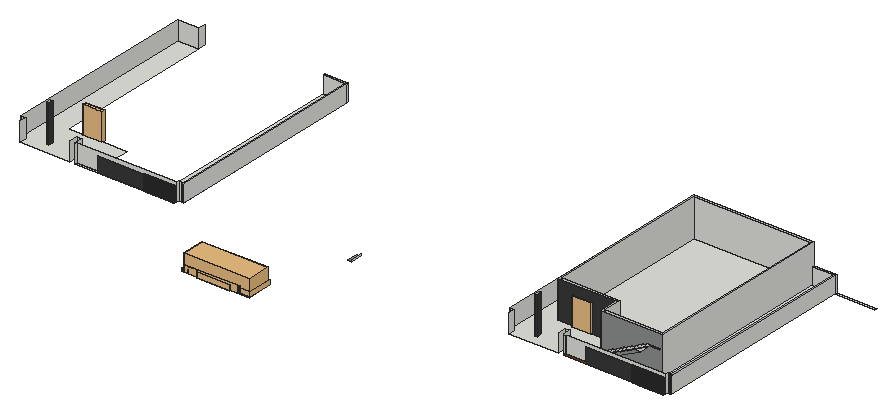
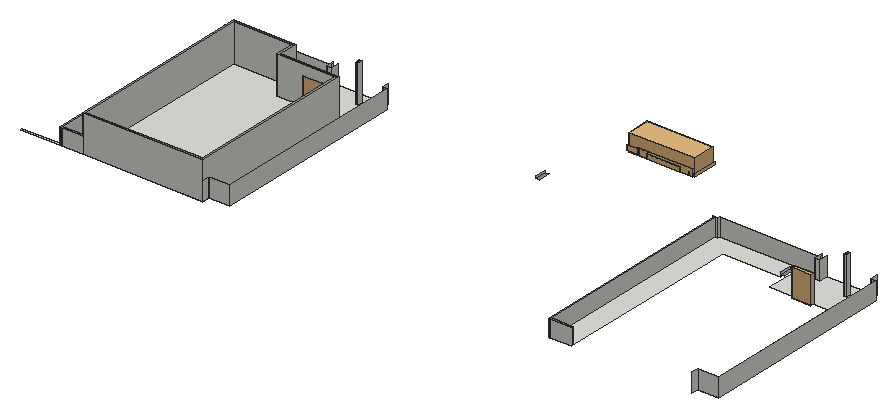
# SketchUp Ruby script. Lengths in inches.
U = 1.inch
M = Sketchup.active_model
def pt(a) = Geom::Point3d.new(a.map { |v| v * U })
def face(e, loops, mat)
  f = e.add_face(loops[0].map { |a| pt(a) })
  loops[1..].each { |l| e.add_face(l.map { |a| pt(a) }).erase! }
  f.material = f.back_material = mat if mat
  f
end
# faces: each face lists its corners as indices into pts; further lists are holes
def faces(e, pts, list, mat = nil) = list.each { |f| face(e, (f[0].is_a?(Array) ? f : [f]).map { |l| l.map { |i| pts[i] } }, mat) }
# xy, xz, yz: faces in a plane at the given z, y or x. An outline is a flat list of corners, or four numbers for a rectangle; further outlines are holes
def ring(l) = l.size == 4 ? [[l[0], l[1]], [l[2], l[1]], [l[2], l[3]], [l[0], l[3]]] : l.each_slice(2).to_a
def flat(e, list, mat, &to3) = list.each { |f| face(e, (f[0].is_a?(Array) ? f : [f]).map { |l| ring(l).map { |u, v| to3.(u, v) } }, mat) }
def xy(e, z, list, mat = nil) = flat(e, list, mat) { |x, y| [x, y, z] }
def xz(e, y, list, mat = nil) = flat(e, list, mat) { |x, z| [x, y, z] }
def yz(e, x, list, mat = nil) = flat(e, list, mat) { |y, z| [x, y, z] }
def lines(e, pts, list) = list.each { |a, b| e.add_line(pt(pts[a]), pt(pts[b])) }
# prism: a flat outline (further loops are holes) pulled along v
def prism(e, loops, v, mat = nil)
  f = face(e, loops, mat); d = Geom::Vector3d.new(v.map { |x| x * U })
  f.pushpull(f.normal.samedirection?(d) ? d.length : -d.length)
end
def box(e, o, s, mat = nil) = prism(e, [[o, [o[0] + s[0], o[1], o[2]], [o[0] + s[0], o[1] + s[1], o[2]], [o[0], o[1] + s[1], o[2]]]], [0, 0, s[2]], mat)
def at(x, y, z, deg = 0) = Geom::Transformation.translation(pt([x, y, z])) * Geom::Transformation.rotation(ORIGIN, Z_AXIS, deg.degrees)
def axes(o, x, y, z) = Geom::Transformation.new([*x, 0, *y, 0, *z, 0, *pt(o).to_a, 1])
def part(name) = M.definitions.add(name)
# library, detail: a bought-in or finely detailed component or shape, given as its bounding box
def library(name, o, s) = part(name).tap { |d| box(d.entities, o, s) }
def detail(e, o, s) = box(e.add_group.entities, o, s)
def put(e, d, t, mat = nil) = e.add_instance(d, t).tap { |i| i.material = mat if mat }
def group(e, t, mat = nil) = e.add_group.tap { |g| g.transformation = t; g.material = mat if mat }.entities
root = M.entities
M.materials.add("[Blacktop Old 02]").color = [143, 145, 145]
M.materials.add("[Color M07]").color = [58, 58, 58]
M.materials.add("[Wood Veneer 01]").color = [120, 70, 37]
M.materials.add("s600").color = [22, 22, 22]
c1 = library("door (1)",[38.93,25.48,0],[40,9.94,82.68])
c2 = library("Group\#542",[3.69,3.66,0],[191.53,68.02,49.26])
c3 = library("Group\#537",[0,0,0],[105.78,6.21,15.76])
c4 = library("Group\#518",[0,0.23,0],[177.37,78.25,22.11])
c5 = library("Group\#530",[0,0,0],[20.12,77.4,9.12])
c6 = library("Group\#533",[0,0,0],[37.78,78.39,15.5])
xy(root,5.875,[[1229.53,300.25,1232.01,301],[1232.72,300.25,1235.19,301],[1235.91,300.25,1238.38,301],[1239.1,300.25,1241.57,301],[1242.28,300.25,1244.76,301],
  [1245.47,300.25,1247.94,301],[1248.66,300.25,1251.13,301],[1251.85,300.25,1254.32,301],[1255.03,300.25,1257.51,301],[1258.22,300.25,1260.69,301],
  [1261.41,300.25,1263.88,301],[1280.53,300.25,1283.01,301],[1283.72,300.25,1286.19,301],[1286.85,300.25,1289.32,301],[1289.97,300.25,1292.44,301],
  [1293.1,300.25,1295.57,301],[1296.22,300.25,1298.69,301],[1299.35,300.25,1301.82,301],[1302.47,300.25,1304.94,301],[1305.6,300.25,1308.07,301],
  [1308.72,300.25,1311.19,301],[1311.85,300.25,1314.32,301],[1314.97,300.25,1317.44,301],[1318.1,300.25,1320.28,301],[2783.53,300.25,2786.01,301],
  [2786.72,300.25,2789.19,301],[2789.91,300.25,2792.38,301],[2793.1,300.25,2795.57,301],[2796.28,300.25,2798.76,301],[2799.47,300.25,2801.94,301],
  [2802.66,300.25,2805.13,301],[2805.85,300.25,2808.32,301],[2809.03,300.25,2811.51,301],[2812.22,300.25,2814.69,301],[2815.41,300.25,2817.88,301],
  [2818.6,300.25,2821.07,301],[2821.78,300.25,2824.26,301],[2824.97,300.25,2827.44,301],[2828.16,300.25,2830.63,301],[2831.35,300.25,2833.82,301],
  [2834.53,300.25,2837.01,301],[2837.72,300.25,2840.19,301],[2840.91,300.25,2843.38,301],[2844.1,300.25,2846.57,301],[2847.28,300.25,2849.76,301],
  [2850.47,300.25,2852.94,301],[2853.6,300.25,2856.07,301],[2856.72,300.25,2859.19,301],[2859.85,300.25,2862.32,301],[2862.97,300.25,2865.44,301],
  [2866.1,300.25,2868.57,301],[2869.22,300.25,2871.69,301],[2872.35,300.25,2874.82,301],[2875.47,300.25,2877.94,301],[2878.6,300.25,2881.07,301],
  [2881.72,300.25,2884.19,301],[2884.85,300.25,2887.03,301],[[823.45,301,982.13,301,982.13,327.09,998.26,327.09,998.26,308.75,1320.28,308.75,1320.28,315.3125,1328.59,315.3125,1328.59,969.375,1260.59,969.375,1260.59,371.33,1072.95,371.33,1072.95,335.33,1061.03,335.33,1061.03,431.33,983.8,431.33,983.8,440.27,922.05,440.27,922.05,431.33,874.71,431.33,874.71,952.09,808.46,952.09,808.46,321.97,823.45,321.97],[879.98,334.62,887.35,350.3]],[998.26,301,1320.28,308.75],[[2390.2,301,2548.88,301,2548.88,327.09,2565.01,327.09,2565.01,308.75,2887.03,308.75,2887.03,315.3125,2895.34,315.3125,2895.34,969.375,2827.34,969.375,2827.34,371.33,2639.7,371.33,2639.7,335.33,2627.78,335.33,2627.78,431.33,2550.55,431.33,2550.55,440.27,2488.8,440.27,2488.8,431.33,2441.46,431.33,2441.46,952.09,2375.21,952.09,2375.21,321.97,2390.2,321.97],[2446.73,334.62,2454.1,350.3]],
  [2565.01,301,2887.03,308.75],[1328.59,315.3125,1334.59,969.375],[2895.34,315.3125,2901.34,969.375],[2627.78,335.33,2627.78,431.33,2550.55,431.33,2550.55,440.27,2633.78,440.27,2633.78,379.21,2822.07,379.21,2822.07,970.67,2446.73,970.67,2446.73,440.27,2488.8,440.27,2488.8,431.33,2441.46,431.33,2441.46,975.9375,2827.34,975.9375,2827.34,371.33,2639.7,371.33,2639.7,335.33],[2633.78,379.21,2822.07,379.21,2822.07,970.67,2446.73,970.67,2446.73,440.27,2633.78,440.27],
  [1260.59,969.375,1328.59,975.9375],[1328.59,969.375,1334.59,975.9375],[2827.34,969.375,2895.34,975.9375],[2895.34,969.375,2901.34,975.9375],[2901.34,969.375,3027.59,975.9375]])
xy(root,11.875,[[1061.03,335.33,1073.03,371.33],[1847.4,335.33,1859.4,371.33],[2627.78,335.33,2639.78,371.33]],"[Blacktop Old 02]")
xz(root,300.25,[[1229.53,5.875,1232.01,54.66],[1232.72,5.875,1235.19,54.66],[1235.91,5.875,1238.38,54.66],[1239.1,5.875,1241.57,54.66],[1242.28,5.875,1244.76,54.66],
  [1245.47,5.875,1247.94,54.66],[1248.66,5.875,1251.13,54.66],[1251.85,5.875,1254.32,54.66],[1255.03,5.875,1257.51,54.66],[1258.22,5.875,1260.69,54.66],
  [1261.41,5.875,1263.88,54.66],[1280.53,5.875,1283.01,54.66],[1283.72,5.875,1286.19,54.66],[1286.85,5.875,1289.32,54.66],[1289.97,5.875,1292.44,54.66],
  [1293.1,5.875,1295.57,54.66],[1296.22,5.875,1298.69,54.66],[1299.35,5.875,1301.82,54.66],[1302.47,5.875,1304.94,54.66],[1305.6,5.875,1308.07,54.66],
  [1308.72,5.875,1311.19,54.66],[1311.85,5.875,1314.32,54.66],[1314.97,5.875,1317.44,54.66],[1318.1,5.875,1320.28,54.66],[2783.53,5.875,2786.01,54.66],
  [2786.72,5.875,2789.19,54.66],[2789.91,5.875,2792.38,54.66],[2793.1,5.875,2795.57,54.66],[2796.28,5.875,2798.76,54.66],[2799.47,5.875,2801.94,54.66],
  [2802.66,5.875,2805.13,54.66],[2805.85,5.875,2808.32,54.66],[2809.03,5.875,2811.51,54.66],[2812.22,5.875,2814.69,54.66],[2815.41,5.875,2817.88,54.66],
  [2818.6,5.875,2821.07,54.66],[2821.78,5.875,2824.26,54.66],[2824.97,5.875,2827.44,54.66],[2828.16,5.875,2830.63,54.66],[2831.35,5.875,2833.82,54.66],
  [2834.53,5.875,2837.01,54.66],[2837.72,5.875,2840.19,54.66],[2840.91,5.875,2843.38,54.66],[2844.1,5.875,2846.57,54.66],[2847.28,5.875,2849.76,54.66],
  [2850.47,5.875,2852.94,54.66],[2853.6,5.875,2856.07,54.66],[2856.72,5.875,2859.19,54.66],[2859.85,5.875,2862.32,54.66],[2862.97,5.875,2865.44,54.66],
  [2866.1,5.875,2868.57,54.66],[2869.22,5.875,2871.69,54.66],[2872.35,5.875,2874.82,54.66],[2875.47,5.875,2877.94,54.66],[2878.6,5.875,2881.07,54.66],
  [2881.72,5.875,2884.19,54.66],[2884.85,5.875,2887.03,54.66]],"[Color M07]")
xz(root,301,[[2887.03,5.875,2887.32,54.66]])
xz(root,301,[[1070.49,5.875,1216.78,54.66],[1219.26,5.875,1219.97,54.66],[1222.44,5.875,1223.16,54.66],[1225.63,5.875,1226.35,54.66],[1228.82,5.875,1229.53,54.66],
  [1232.01,5.875,1232.72,54.66],[1235.19,5.875,1235.91,54.66],[1238.38,5.875,1239.1,54.66],[1241.57,5.875,1242.28,54.66],[1244.76,5.875,1245.47,54.66],
  [1247.94,5.875,1248.66,54.66],[1251.13,5.875,1251.85,54.66],[1254.32,5.875,1255.03,54.66],[1257.51,5.875,1258.22,54.66],[1260.69,5.875,1261.41,54.66],
  [1263.88,5.875,1264.6,54.66],[1267.07,5.875,1267.78,54.66],[1270.26,5.875,1270.97,54.66],[1273.44,5.875,1274.16,54.66],[1276.63,5.875,1277.35,54.66],
  [1279.82,5.875,1280.53,54.66],[1317.44,5.875,1318.1,54.66],[2637.24,5.875,2783.53,54.66],[2786.01,5.875,2786.72,54.66],[2789.19,5.875,2789.91,54.66],
  [2792.38,5.875,2793.1,54.66],[2795.57,5.875,2796.28,54.66],[2798.76,5.875,2799.47,54.66],[2801.94,5.875,2802.66,54.66],[2805.13,5.875,2805.85,54.66],
  [2808.32,5.875,2809.03,54.66],[2811.51,5.875,2812.22,54.66],[2814.69,5.875,2815.41,54.66],[2817.88,5.875,2818.6,54.66],[2821.07,5.875,2821.78,54.66],
  [2824.26,5.875,2824.97,54.66],[2827.44,5.875,2828.16,54.66],[2830.63,5.875,2831.35,54.66],[2833.82,5.875,2834.53,54.66],[2837.01,5.875,2837.72,54.66],
  [2840.19,5.875,2840.91,54.66],[2843.38,5.875,2844.1,54.66],[2846.57,5.875,2847.28,54.66],[2849.76,5.875,2850.47,54.66],[2852.94,5.875,2853.6,54.66],
  [2856.07,5.875,2856.72,54.66],[2859.19,5.875,2859.85,54.66],[2862.32,5.875,2862.97,54.66],[2865.44,5.875,2866.1,54.66],[2868.57,5.875,2869.22,54.66],
  [2871.69,5.875,2872.35,54.66],[2874.82,5.875,2875.47,54.66],[2877.94,5.875,2878.6,54.66],[2881.07,5.875,2881.72,54.66],[2884.19,5.875,2884.85,54.66]],"[Color M07]")
xz(root,301,[[2565.01,5.875,2637.24,13.04]],"[Wood Veneer 01]")
xz(root,308.75,[[998.26,5.875,1320.28,62.25],[2565.01,5.875,2887.03,62.25]])
xz(root,315.3125,[[1320.28,5.875,1320.28,62.25,1334.59,62.25,1334.59,58.8125,1328.59,58.8125,1328.59,5.875],[1328.59,5.875,1334.59,58.8125],[2887.03,5.875,2887.03,62.25,2901.34,62.25,2901.34,58.8125,2895.34,58.8125,2895.34,5.875],[2895.34,5.875,2901.34,58.8125]])
xz(root,321.97,[[808.46,5.875,823.45,65.875],[2375.21,5.875,2390.2,65.875]])
xz(root,327.09,[[982.13,5.875,998.26,65.875],[2548.88,5.875,2565.01,65.875]])
xz(root,334.62,[[879.98,5.875,887.35,125.875],[2446.73,5.875,2454.1,125.875]],"[Color M07]")
xz(root,335.33,[[2627.78,5.875,2639.7,5.875,2783.78,77.875,2759.78,77.875,2759.78,71.875,2747.78,71.875,2747.78,65.875,2735.78,65.875,2735.78,59.875,2723.78,59.875,2723.78,53.875,2711.78,53.875,2711.78,47.875,2699.78,47.875,2699.78,41.875,2687.78,41.875,2687.78,35.875,2675.78,35.875,2675.78,29.875,2663.78,29.875,2663.78,23.875,2651.78,23.875,2651.78,17.875,2639.78,17.875,2639.78,11.875,2627.78,11.875]],"[Blacktop Old 02]")
xz(root,350.3,[[879.98,5.875,887.35,125.875],[2446.73,5.875,2454.1,125.875]])
xz(root,371.33,[[2639.7,5.875,2827.34,5.875,2827.34,125.875,2627.78,125.875,2627.78,11.875,2639.78,11.875,2639.78,17.875,2651.78,17.875,2651.78,23.875,2663.78,23.875,2663.78,29.875,2675.78,29.875,2675.78,35.875,2687.78,35.875,2687.78,41.875,2699.78,41.875,2699.78,47.875,2711.78,47.875,2711.78,53.875,2723.78,53.875,2723.78,59.875,2735.78,59.875,2735.78,65.875,2747.78,65.875,2747.78,71.875,2759.78,71.875,2759.78,77.875,2771.78,77.875,2771.78,83.875,2819.78,83.875,2819.78,77.875,2783.78,77.875]],"[Blacktop Old 02]")
xz(root,379.21,[[2633.78,5.875,2822.07,125.875]])
xz(root,431.33,[[2441.46,5.875,2488.8,5.875,2488.8,94.0625,2550.55,94.0625,2550.55,5.875,2627.78,5.875,2627.78,125.875,2441.46,125.875]],"[Color M07]")
xz(root,440.27,[[2446.73,5.875,2446.73,125.875,2633.78,125.875,2633.78,5.875,2550.55,5.875,2550.55,94.0625,2488.8,94.0625,2488.8,5.875]])
xz(root,952.09,[[808.46,5.875,874.71,65.875],[2375.21,5.875,2441.46,65.875]])
xz(root,969.375,[[1260.59,5.875,1328.59,58.8125],[1328.59,5.875,1334.59,58.8125],[2827.34,5.875,2895.34,58.8125],[2895.34,5.875,2901.34,58.8125]])
xz(root,970.67,[[2446.73,5.875,2822.07,125.875]])
xz(root,975.9375,[[1260.59,5.875,1328.59,58.8125],[1328.59,5.875,1334.59,58.8125],[2441.46,5.875,2827.34,125.875],[2827.34,5.875,2895.34,58.8125],[2895.34,5.875,2901.34,58.8125]])
yz(root,808.46,[[321.97,5.875,952.09,65.875]])
yz(root,823.45,[[301,5.875,321.97,65.875]])
yz(root,874.71,[[952.09,5.875,975.9375,65.875]])
yz(root,879.98,[[334.62,5.875,350.3,125.875]])
yz(root,887.35,[[334.62,5.875,350.3,125.875]],"[Color M07]")
yz(root,982.13,[[301,5.875,327.09,65.875]])
yz(root,998.26,[[301,5.875,308.75,62.25],[308.75,5.875,327.09,5.875,327.09,65.875,301,65.875,301,62.25,308.75,62.25]])
yz(root,1073.03,[[335.33,11.875,371.33,17.875]])
yz(root,1229.53,[[300.25,5.875,301,54.66]])
yz(root,1232.01,[[300.25,5.875,301,54.66]])
yz(root,1232.72,[[300.25,5.875,301,54.66]])
yz(root,1235.19,[[300.25,5.875,301,54.66]])
yz(root,1235.91,[[300.25,5.875,301,54.66]])
yz(root,1238.38,[[300.25,5.875,301,54.66]])
yz(root,1239.1,[[300.25,5.875,301,54.66]])
yz(root,1241.57,[[300.25,5.875,301,54.66]])
yz(root,1242.28,[[300.25,5.875,301,54.66]])
yz(root,1244.76,[[300.25,5.875,301,54.66]])
yz(root,1245.47,[[300.25,5.875,301,54.66]])
yz(root,1247.94,[[300.25,5.875,301,54.66]])
yz(root,1248.66,[[300.25,5.875,301,54.66]])
yz(root,1251.13,[[300.25,5.875,301,54.66]])
yz(root,1251.85,[[300.25,5.875,301,54.66]])
yz(root,1254.32,[[300.25,5.875,301,54.66]])
yz(root,1255.03,[[300.25,5.875,301,54.66]])
yz(root,1257.51,[[300.25,5.875,301,54.66]])
yz(root,1258.22,[[300.25,5.875,301,54.66]])
yz(root,1260.69,[[300.25,5.875,301,54.66]])
yz(root,1261.41,[[300.25,5.875,301,54.66]])
yz(root,1263.88,[[300.25,5.875,301,54.66]])
yz(root,1277.35,[[300.25,5.875,301,54.66]])
yz(root,1280.53,[[300.25,5.875,301,54.66]])
yz(root,1283.01,[[300.25,5.875,301,54.66]])
yz(root,1283.72,[[300.25,5.875,301,54.66]])
yz(root,1286.19,[[300.25,5.875,301,54.66]])
yz(root,1286.85,[[300.25,5.875,301,54.66]])
yz(root,1289.32,[[300.25,5.875,301,54.66]])
yz(root,1289.97,[[300.25,5.875,301,54.66]])
yz(root,1292.44,[[300.25,5.875,301,54.66]])
yz(root,1293.1,[[300.25,5.875,301,54.66]])
yz(root,1295.57,[[300.25,5.875,301,54.66]])
yz(root,1296.22,[[300.25,5.875,301,54.66]])
yz(root,1298.69,[[300.25,5.875,301,54.66]])
yz(root,1302.47,[[300.25,5.875,301,54.66]])
yz(root,1311.19,[[300.25,5.875,301,54.66]])
yz(root,1311.85,[[300.25,5.875,301,54.66]])
yz(root,1314.32,[[300.25,5.875,301,54.66]])
yz(root,1314.97,[[300.25,5.875,301,54.66]])
yz(root,1317.44,[[300.25,5.875,301,54.66]])
yz(root,1318.1,[[300.25,5.875,301,54.66]])
yz(root,1320.28,[[300.25,5.875,301,54.66],[308.75,5.875,315.3125,62.25]])
yz(root,1328.59,[[315.3125,5.875,969.375,58.8125],[969.375,5.875,975.9375,58.8125]])
yz(root,1334.59,[[315.3125,5.875,969.375,58.8125],[969.375,5.875,975.9375,58.8125]])
yz(root,1859.4,[[335.33,11.875,371.33,17.875]])
yz(root,2375.21,[[321.97,5.875,952.09,65.875]])
yz(root,2390.2,[[301,5.875,321.97,65.875]])
yz(root,2441.46,[[431.33,5.875,431.33,125.875,975.9375,125.875,975.9375,65.875,952.09,65.875,952.09,5.875],[952.09,5.875,975.9375,65.875]])
yz(root,2446.73,[[334.62,5.875,350.3,125.875],[440.27,5.875,970.67,125.875]])
yz(root,2454.1,[[334.62,5.875,350.3,125.875]],"[Color M07]")
yz(root,2488.8,[[431.33,5.875,440.27,94.0625]])
yz(root,2548.88,[[301,5.875,327.09,65.875]])
yz(root,2550.55,[[431.33,5.875,440.27,94.0625]])
yz(root,2565.01,[[301,5.875,308.75,62.25],[308.75,5.875,327.09,5.875,327.09,65.875,301,65.875,301,62.25,308.75,62.25]])
yz(root,2627.78,[[335.33,5.875,335.33,11.875,371.33,11.875,371.33,125.875,431.33,125.875,431.33,5.875]])
yz(root,2633.78,[[379.21,5.875,440.27,125.875]])
yz(root,2639.78,[[335.33,11.875,371.33,17.875]])
yz(root,2783.53,[[300.25,5.875,301,54.66]])
yz(root,2786.01,[[300.25,5.875,301,54.66]])
yz(root,2786.72,[[300.25,5.875,301,54.66]])
yz(root,2789.19,[[300.25,5.875,301,54.66]])
yz(root,2789.91,[[300.25,5.875,301,54.66]])
yz(root,2792.38,[[300.25,5.875,301,54.66]])
yz(root,2793.1,[[300.25,5.875,301,54.66]])
yz(root,2795.57,[[300.25,5.875,301,54.66]])
yz(root,2796.28,[[300.25,5.875,301,54.66]])
yz(root,2798.76,[[300.25,5.875,301,54.66]])
yz(root,2799.47,[[300.25,5.875,301,54.66]])
yz(root,2801.94,[[300.25,5.875,301,54.66]])
yz(root,2802.66,[[300.25,5.875,301,54.66]])
yz(root,2805.13,[[300.25,5.875,301,54.66]])
yz(root,2805.85,[[300.25,5.875,301,54.66]])
yz(root,2808.32,[[300.25,5.875,301,54.66]])
yz(root,2809.03,[[300.25,5.875,301,54.66]])
yz(root,2811.51,[[300.25,5.875,301,54.66]])
yz(root,2812.22,[[300.25,5.875,301,54.66]])
yz(root,2814.69,[[300.25,5.875,301,54.66]])
yz(root,2815.41,[[300.25,5.875,301,54.66]])
yz(root,2817.88,[[300.25,5.875,301,54.66]])
yz(root,2818.6,[[300.25,5.875,301,54.66]])
yz(root,2821.07,[[300.25,5.875,301,54.66]])
yz(root,2821.78,[[300.25,5.875,301,54.66]])
yz(root,2822.07,[[379.21,5.875,970.67,125.875]])
yz(root,2824.26,[[300.25,5.875,301,54.66]])
yz(root,2824.97,[[300.25,5.875,301,54.66]])
yz(root,2827.34,[[371.33,5.875,969.375,5.875,969.375,58.8125,975.9375,58.8125,975.9375,125.875,371.33,125.875]])
yz(root,2827.44,[[300.25,5.875,301,54.66]])
yz(root,2828.16,[[300.25,5.875,301,54.66]])
yz(root,2830.63,[[300.25,5.875,301,54.66]])
yz(root,2831.35,[[300.25,5.875,301,54.66]])
yz(root,2833.82,[[300.25,5.875,301,54.66]])
yz(root,2834.53,[[300.25,5.875,301,54.66]])
yz(root,2837.01,[[300.25,5.875,301,54.66]])
yz(root,2837.72,[[300.25,5.875,301,54.66]])
yz(root,2840.19,[[300.25,5.875,301,54.66]])
yz(root,2840.91,[[300.25,5.875,301,54.66]])
yz(root,2843.38,[[300.25,5.875,301,54.66]])
yz(root,2844.1,[[300.25,5.875,301,54.66]])
yz(root,2846.57,[[300.25,5.875,301,54.66]])
yz(root,2847.28,[[300.25,5.875,301,54.66]])
yz(root,2849.76,[[300.25,5.875,301,54.66]])
yz(root,2850.47,[[300.25,5.875,301,54.66]])
yz(root,2852.94,[[300.25,5.875,301,54.66]])
yz(root,2853.6,[[300.25,5.875,301,54.66]])
yz(root,2856.07,[[300.25,5.875,301,54.66]])
yz(root,2856.72,[[300.25,5.875,301,54.66]])
yz(root,2859.19,[[300.25,5.875,301,54.66]])
yz(root,2859.85,[[300.25,5.875,301,54.66]])
yz(root,2862.32,[[300.25,5.875,301,54.66]])
yz(root,2862.97,[[300.25,5.875,301,54.66]])
yz(root,2865.44,[[300.25,5.875,301,54.66]])
yz(root,2866.1,[[300.25,5.875,301,54.66]])
yz(root,2868.57,[[300.25,5.875,301,54.66]])
yz(root,2869.22,[[300.25,5.875,301,54.66]])
yz(root,2871.69,[[300.25,5.875,301,54.66]])
yz(root,2872.35,[[300.25,5.875,301,54.66]])
yz(root,2874.82,[[300.25,5.875,301,54.66]])
yz(root,2875.47,[[300.25,5.875,301,54.66]])
yz(root,2877.94,[[300.25,5.875,301,54.66]])
yz(root,2878.6,[[300.25,5.875,301,54.66]])
yz(root,2881.07,[[300.25,5.875,301,54.66]])
yz(root,2881.72,[[300.25,5.875,301,54.66]])
yz(root,2884.19,[[300.25,5.875,301,54.66]])
yz(root,2884.85,[[300.25,5.875,301,54.66]])
yz(root,2887.03,[[300.25,5.875,301,54.66],[308.75,5.875,315.3125,62.25]])
yz(root,2895.34,[[315.3125,5.875,969.375,58.8125],[969.375,5.875,975.9375,58.8125]])
yz(root,2901.34,[[315.3125,5.875,969.375,58.8125],[969.375,5.875,975.9375,58.8125]])
p = [[2639.7,371.33,5.875],[2783.78,371.33,77.875],[2783.78,335.33,77.875],[2639.7,335.33,5.875]]
faces(root,p,[[0,1,2,3]])
put(root,c1,axes([861.96,403.11,5.875],[1.54375,0,0],[0,1,0],[0,0,1.06665]))
put(root,c1,axes([2428.71,403.11,5.875],[1.54375,0,0],[0,1,0],[0,0,1.06665]))
put(root,c2,axes([1553.33,116.78,7.08],[1.10376,0,0],[0,-1.10376,0],[0,0,1.10376]))
put(root,c3,at(1601.96,109.08,7.79),"s600")
put(root,c4,at(1560.23,35.85,7.79),"s600")
put(root,c3,axes([1601.96,41.32,7.79],[1,0,0],[0,-1,0],[0,0,1]),"s600")
put(root,c5,at(1553.39,36.5,9.8),"s600")
put(root,c6,at(1733.23,36.01,10.8125),"s600")
